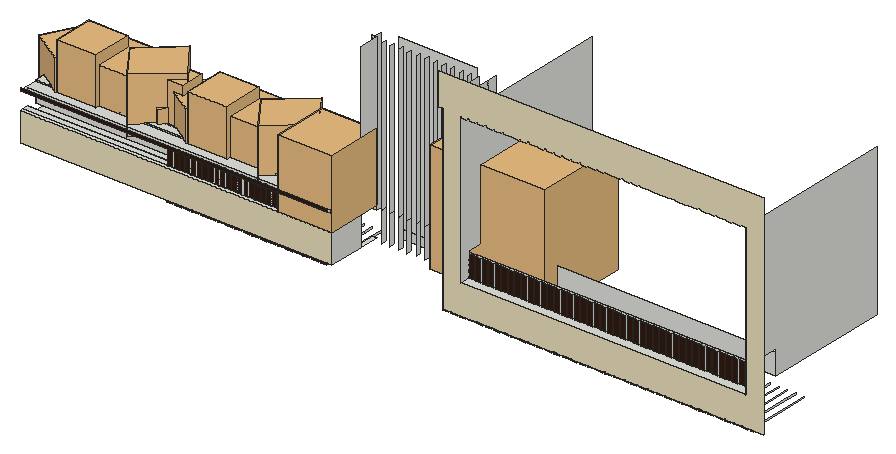
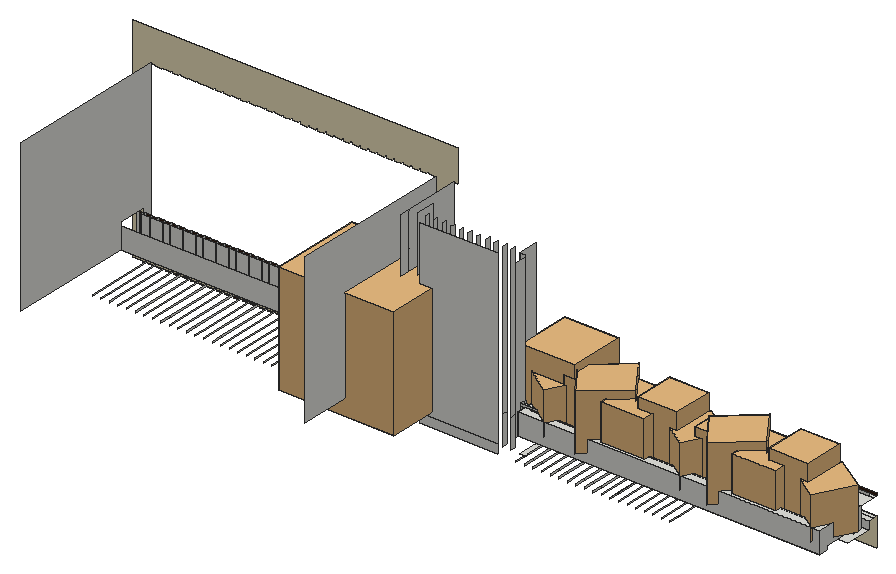
# SketchUp Ruby script. Lengths in inches.
U = 1.inch
M = Sketchup.active_model
def pt(a) = Geom::Point3d.new(a.map { |v| v * U })
def face(e, loops, mat)
  f = e.add_face(loops[0].map { |a| pt(a) })
  loops[1..].each { |l| e.add_face(l.map { |a| pt(a) }).erase! }
  f.material = f.back_material = mat if mat
  f
end
# faces: each face lists its corners as indices into pts; further lists are holes
def faces(e, pts, list, mat = nil) = list.each { |f| face(e, (f[0].is_a?(Array) ? f : [f]).map { |l| l.map { |i| pts[i] } }, mat) }
# xy, xz, yz: faces in a plane at the given z, y or x. An outline is a flat list of corners, or four numbers for a rectangle; further outlines are holes
def ring(l) = l.size == 4 ? [[l[0], l[1]], [l[2], l[1]], [l[2], l[3]], [l[0], l[3]]] : l.each_slice(2).to_a
def flat(e, list, mat, &to3) = list.each { |f| face(e, (f[0].is_a?(Array) ? f : [f]).map { |l| ring(l).map { |u, v| to3.(u, v) } }, mat) }
def xy(e, z, list, mat = nil) = flat(e, list, mat) { |x, y| [x, y, z] }
def xz(e, y, list, mat = nil) = flat(e, list, mat) { |x, z| [x, y, z] }
def yz(e, x, list, mat = nil) = flat(e, list, mat) { |y, z| [x, y, z] }
def lines(e, pts, list) = list.each { |a, b| e.add_line(pt(pts[a]), pt(pts[b])) }
# prism: a flat outline (further loops are holes) pulled along v
def prism(e, loops, v, mat = nil)
  f = face(e, loops, mat); d = Geom::Vector3d.new(v.map { |x| x * U })
  f.pushpull(f.normal.samedirection?(d) ? d.length : -d.length)
end
def box(e, o, s, mat = nil) = prism(e, [[o, [o[0] + s[0], o[1], o[2]], [o[0] + s[0], o[1] + s[1], o[2]], [o[0], o[1] + s[1], o[2]]]], [0, 0, s[2]], mat)
def at(x, y, z, deg = 0) = Geom::Transformation.translation(pt([x, y, z])) * Geom::Transformation.rotation(ORIGIN, Z_AXIS, deg.degrees)
def axes(o, x, y, z) = Geom::Transformation.new([*x, 0, *y, 0, *z, 0, *pt(o).to_a, 1])
def part(name) = M.definitions.add(name)
# library, detail: a bought-in or finely detailed component or shape, given as its bounding box
def library(name, o, s) = part(name).tap { |d| box(d.entities, o, s) }
def detail(e, o, s) = box(e.add_group.entities, o, s)
def put(e, d, t, mat = nil) = e.add_instance(d, t).tap { |i| i.material = mat if mat }
def group(e, t, mat = nil) = e.add_group.tap { |g| g.transformation = t; g.material = mat if mat }.entities
root = M.entities
M.materials.add("Material__1").color = [95, 70, 46]
M.materials.add("[Color D01]").color = [237, 225, 189]
M.materials.add("[Wood Veneer 01]").color = [51, 28, 15]
c1 = library("Areca palm plant",[0,0,0],[49.1,36.6,54.46])
c2 = library("Group\#74",[-84.69,-90.07,-0.36],[176.51,175.13,171.4])
c3 = library("Group20\#1",[-20.81,-17.08,3.79],[39.86,39.43,37.51])
c4 = library("Group\#130",[-7.34,-1.2,0],[38.67,35.81,49.04])
c5 = library("Group38\#2",[14.01,28.44,-23.43],[18.58,18.32,38.89])
c6 = part("Group\#16")
put(c6.entities,c1,axes([-6.2,158.41,6.08],[0.45017,-0.56191,0],[0.66137,0.52986,0],[0,0,0.72]))
put(c6.entities,c1,axes([-6.2,56.6,6.08],[0.45017,-0.56191,0],[0.66137,0.52986,0],[0,0,0.72]))
put(c6.entities,c2,axes([14.93,145.87,6.05],[-0.04961,-0.08593,0],[0.08593,-0.04961,0],[0,0,0.10522]))
put(c6.entities,c3,axes([18.97,79.98,4.77],[0,0.85,0],[-0.85,0,0],[0,0,0.85]))
put(c6.entities,c2,axes([14.93,173.12,6.05],[-0.04961,-0.08593,0],[0.08593,-0.04961,0],[0,0,0.10522]))
put(c6.entities,c2,axes([14.93,193.18,6.05],[-0.04961,-0.08593,0],[0.08593,-0.04961,0],[0,0,0.10522]))
put(c6.entities,c4,axes([24.9375,89.91,8],[0,0.79,0],[-0.79,0,0],[0,0,0.79]))
put(c6.entities,c5,axes([-4.1,-1.15,28.17],[0.8848,0,0],[0,0.94674,0],[0,0,0.85826]))
g1 = group(c6.entities,at(0,0,0))
xy(g1,0,[[0,0,6,234.8],[30,0,36,234.8]])
xy(g1,3,[[6,0,30,234.8]])
xy(g1,7,[[6,5,30,229.8]],"Material__1")
xy(g1,15,[[[0,0,36,234.8],[6,5,30,229.8]]])
xz(g1,0,[[0,0,6,0,6,3,30,3,30,0,36,0,36,15,0,15]])
xz(g1,5,[[6,7,30,15]])
xz(g1,229.8,[[6,7,30,15]])
xz(g1,234.8,[[0,0,0,15,36,15,36,0,30,0,30,3,6,3,6,0]])
yz(g1,0,[[0,0,234.8,15]])
yz(g1,6,[[0,0,234.8,3],[5,7,229.8,15]])
yz(g1,30,[[0,0,234.8,3],[5,7,229.8,15]])
yz(g1,36,[[0,0,234.8,15]])
put(c6.entities,c2,axes([14.93,91.37,6.05],[-0.04961,-0.08593,0],[0.08593,-0.04961,0],[0,0,0.10522]))
put(c6.entities,c2,axes([14.93,44.05,6.05],[-0.04961,-0.08593,0],[0.08593,-0.04961,0],[0,0,0.10522]))
put(c6.entities,c4,axes([24.9375,191.72,8],[0,0.79,0],[-0.79,0,0],[0,0,0.79]))
put(c6.entities,c5,axes([-4.1,100.66,28.17],[0.8848,0,0],[0,0.94674,0],[0,0,0.85826]))
put(c6.entities,c2,axes([17.19,15.79,6.07],[-0.08133,-0.14087,0],[0.14087,-0.08133,0],[0,0,0.1725]))
put(c6.entities,c2,axes([14.93,71.3,6.05],[-0.04961,-0.08593,0],[0.08593,-0.04961,0],[0,0,0.10522]))
put(c6.entities,c2,axes([17.19,121.23,6.07],[-0.08133,-0.14087,0],[0.14087,-0.08133,0],[0,0,0.1725]))
put(c6.entities,c2,axes([17.19,223.04,6.07],[-0.08133,-0.14087,0],[0.14087,-0.08133,0],[0,0,0.1725]))
put(c6.entities,c3,axes([18.97,181.79,4.77],[0,0.85,0],[-0.85,0,0],[0,0,0.85]))
c7 = library("plant (1)",[-35.72,-28.42,0],[66.31,67.39,84.38])
c8 = library("Round Planter with Plant",[-35.48,-39.77,0],[80.62,63.55,77.875])
xy(root,254.6875,[[1782.56,246.64,1785.93,286.21]])
xy(root,269.0625,[[1567.3,253.58,1567.3,271.8,1769.03,271.8,1769.03,290.02,1776.11,290.02,1776.11,253.58]])
xy(root,275.125,[[1567.3,246.64,1785.93,249.27],[1876.45,246.64,2076.2,246.64,2076.2,255.84,1880.14,255.84,1880.14,253.84,1876.45,253.84],[1567.3,249.27,1782.56,253.58],[1782.56,249.27,1785.93,253.58],[1776.11,253.58,1782.56,290.02],
  [1782.56,253.58,1785.93,286.21],[1876.45,253.84,1880.14,255.47]])
xy(root,287.25,[[1567.3,246.64,1782.56,249.27],[1782.56,246.64,1785.1875,249.27],[1567.3,249.27,1567.3,271.8,1769.03,271.8,1769.03,290.02,1782.56,290.02,1782.56,249.27],[1782.56,249.27,1785.1875,286.21]])
xz(root,246.64,[[1711.81,254.625,1716.56,254.6875],[1782.56,287.25,1785.1875,289.1875]])
xz(root,246.64,[[1567.3,254.6875,1785.93,275.125],[[1863.7,254.6875,2089.125,254.6875,2089.125,403.1875,1861.07,403.1875,1861.07,380.6875,1863.7,380.6875],[1876.45,275.125,1876.45,379.5625,1880.86,379.5625,1880.86,380.6875,1882.45,380.6875,1882.45,379.5625,1886.86,379.5625,1886.86,380.6875,1888.45,380.6875,1888.45,379.5625,1892.86,379.5625,1892.86,380.6875,1894.45,380.6875,1894.45,379.5625,1898.86,379.5625,1898.86,380.6875,1900.45,380.6875,1900.45,379.5625,1904.86,379.5625,1904.86,380.6875,1906.45,380.6875,1906.45,379.5625,1910.86,379.5625,1910.86,380.6875,1912.45,380.6875,1912.45,379.5625,1916.86,379.5625,1916.86,380.6875,1918.45,380.6875,1918.45,379.5625,1922.86,379.5625,1922.86,380.6875,1924.45,380.6875,1924.45,379.5625,1928.86,379.5625,1928.86,380.6875,1930.45,380.6875,1930.45,379.5625,1934.86,379.5625,1934.86,380.6875,1936.45,380.6875,1936.45,379.5625,1940.86,379.5625,1940.86,380.6875,1942.45,380.6875,1942.45,379.5625,1946.86,379.5625,1946.86,380.6875,1948.45,380.6875,1948.45,379.5625,1952.86,379.5625,1952.86,380.6875,1954.45,380.6875,1954.45,379.5625,1958.86,379.5625,1958.86,380.6875,1960.45,380.6875,1960.45,379.5625,1964.86,379.5625,1964.86,380.6875,1966.45,380.6875,1966.45,379.5625,1970.86,379.5625,1970.86,380.6875,1972.45,380.6875,1972.45,380.0625,1976.86,380.0625,1976.86,380.6875,1978.45,380.6875,1978.45,380.0625,1982.86,380.0625,1982.86,380.6875,1984.45,380.6875,1984.45,380.0625,1988.86,380.0625,1988.86,380.6875,1990.45,380.6875,1990.45,380.0625,1994.86,380.0625,1994.86,380.6875,1996.45,380.6875,1996.45,380.0625,2000.86,380.0625,2000.86,380.6875,2002.45,380.6875,2002.45,380.0625,2006.86,380.0625,2006.86,380.6875,2008.45,380.6875,2008.45,380.0625,2012.86,380.0625,2012.86,380.6875,2014.45,380.6875,2014.45,380.0625,2018.86,380.0625,2018.86,380.6875,2020.45,380.6875,2020.45,380.0625,2024.86,380.0625,2024.86,380.6875,2026.45,380.6875,2026.45,380.0625,2030.86,380.0625,2030.86,380.6875,2032.45,380.6875,2032.45,380.0625,2036.86,380.0625,2036.86,380.6875,2038.45,380.6875,2038.45,380.1875,2042.86,380.1875,2042.86,380.6875,2044.45,380.6875,2044.45,380.1875,2048.86,380.1875,2048.86,380.6875,2050.45,380.6875,2050.45,380.1875,2054.86,380.1875,2054.86,380.6875,2056.45,380.6875,2056.45,380.1875,2060.86,380.1875,2060.86,380.6875,2062.45,380.6875,2062.45,380.1875,2066.86,380.1875,2066.86,380.6875,2068.45,380.6875,2068.45,380.1875,2072.86,380.1875,2072.86,380.6875,2076.2,380.6875,2076.2,275.125]]],"[Color D01]")
xz(root,246.64,[[1723.81,253.5625,1728.56,254.6875],[1729.81,253.5625,1734.56,254.6875],[1735.81,253.5625,1740.56,254.6875],[1741.81,253.5625,1746.56,254.6875],[1747.81,253.5625,1752.56,254.6875],
  [1753.81,253.5625,1758.56,254.6875],[1759.81,253.5625,1764.56,254.6875],[1765.81,253.5625,1770.56,254.6875],[1771.81,253.5625,1776.56,254.6875],[1777.81,253.5625,1782.56,254.6875],
  [1711.81,253.875,1716.56,254.625],[1717.81,253.875,1722.56,254.6875],[1669.81,253.9375,1674.56,254.6875],[1675.81,253.9375,1680.56,254.6875],[1681.81,253.9375,1686.56,254.6875],
  [1687.81,253.9375,1692.56,254.6875],[1693.81,253.9375,1698.56,254.6875],[1699.81,253.9375,1704.56,254.6875],[1705.81,253.9375,1710.56,254.6875],[1863.7,253.9375,1868.08,254.6875],
  [1869.7,253.9375,1874.08,254.6875],[1875.7,253.9375,1880.08,254.6875],[1881.7,253.9375,1886.08,254.6875],[1887.7,253.9375,1892.08,254.6875],[1893.7,253.9375,1898.08,254.6875],
  [1899.7,253.9375,1904.08,254.6875],[1905.7,253.9375,1910.08,254.6875],[1911.7,253.9375,1916.08,254.6875],[1917.7,253.9375,1922.08,254.6875],[1923.7,253.9375,1928.08,254.6875],
  [1929.7,253.9375,1934.08,254.6875],[1935.7,253.9375,1940.08,254.6875],[1941.7,253.9375,1946.08,254.6875],[1947.7,253.9375,1952.08,254.6875],[1953.7,253.9375,1958.08,254.6875],
  [1959.7,253.9375,1964.08,254.6875],[1965.7,253.9375,1970.08,254.6875],[1971.7,253.9375,1976.08,254.6875],[1977.7,253.9375,1982.08,254.6875],[1983.7,253.9375,1988.08,254.6875],
  [1989.7,253.9375,1994.08,254.6875],[1995.7,253.9375,2000.08,254.6875],[2001.7,253.9375,2006.08,254.6875],[2007.7,253.9375,2012.08,254.6875],[2013.7,253.9375,2018.08,254.6875],
  [2019.7,253.9375,2024.08,254.6875],[2025.7,253.9375,2030.08,254.6875],[2031.7,253.9375,2036.08,254.6875],[2037.7,253.9375,2042.08,254.6875],[2043.7,253.9375,2048.08,254.6875],
  [2049.7,253.9375,2054.08,254.6875],[2055.7,253.9375,2060.08,254.6875],[2061.7,253.9375,2066.08,254.6875],[2067.7,253.9375,2072.08,254.6875],[2073.7,253.9375,2078.08,254.6875],
  [2079.7,253.9375,2081.89,254.6875],[1567.3,287.25,1782.56,289.1875]],"[Wood Veneer 01]")
xz(root,249.27,[[1672.14,275.125,1672.93,287.25],[1676.2,275.125,1676.99,287.25],[1680.27,275.125,1681.05,287.25],[1684.33,275.125,1685.11,287.25],[1688.39,275.125,1689.18,287.25],
  [1692.45,275.125,1693.24,287.25],[1696.52,275.125,1697.3,287.25],[1700.58,275.125,1701.36,287.25],[1704.64,275.125,1705.43,287.25],[1708.7,275.125,1709.49,287.25],
  [1712.77,275.125,1713.55,287.25],[1716.83,275.125,1717.61,287.25],[1720.89,275.125,1721.68,287.25],[1724.95,275.125,1725.74,287.25],[1729.02,275.125,1729.8,287.25],
  [1733.08,275.125,1733.86,287.25],[1737.14,275.125,1737.93,287.25],[1741.2,275.125,1741.99,287.25],[1745.27,275.125,1746.05,287.25],[1749.33,275.125,1750.11,287.25],
  [1753.39,275.125,1754.18,287.25],[1757.45,275.125,1758.24,287.25],[1761.52,275.125,1762.3,287.25],[1765.58,275.125,1766.36,287.25],[1769.64,275.125,1770.43,287.25],
  [1773.7,275.125,1774.49,287.25],[1777.77,275.125,1778.55,287.25],[1781.83,275.125,1782.56,287.25],[1570.58,287.25,1782.56,289.1875],[1782.56,287.25,1785.1875,289.1875]])
xz(root,249.27,[[1668.86,275.125,1672.14,287.25],[1672.93,275.125,1676.2,287.25],[1676.99,275.125,1680.27,287.25],[1681.05,275.125,1684.33,287.25],[1685.11,275.125,1688.39,287.25],
  [1689.18,275.125,1692.45,287.25],[1693.24,275.125,1696.52,287.25],[1697.3,275.125,1700.58,287.25],[1701.36,275.125,1704.64,287.25],[1705.43,275.125,1708.7,287.25],
  [1709.49,275.125,1712.77,287.25],[1713.55,275.125,1716.83,287.25],[1717.61,275.125,1720.89,287.25],[1721.68,275.125,1724.95,287.25],[1725.74,275.125,1729.02,287.25],
  [1729.8,275.125,1733.08,287.25],[1733.86,275.125,1737.14,287.25],[1737.93,275.125,1741.2,287.25],[1741.99,275.125,1745.27,287.25],[1746.05,275.125,1749.33,287.25],
  [1750.11,275.125,1753.39,287.25],[1754.18,275.125,1757.45,287.25],[1758.24,275.125,1761.52,287.25],[1762.3,275.125,1765.58,287.25],[1766.36,275.125,1769.64,287.25],
  [1770.43,275.125,1773.7,287.25],[1774.49,275.125,1777.77,287.25],[1778.55,275.125,1781.83,287.25]],"[Wood Veneer 01]")
xz(root,253.58,[[1567.3,269.0625,1776.11,275.125]])
xz(root,253.84,[[1876.45,275.125,1880.14,290.375],[1881.07,275.125,1884.76,290.375],[1885.7,275.125,1889.39,290.375],[1890.32,275.125,1894.01,290.375],[1894.95,275.125,1898.64,290.375],
  [1899.57,275.125,1903.26,290.375],[1904.2,275.125,1907.89,290.375],[1908.82,275.125,1912.51,290.375],[1913.45,275.125,1917.14,290.375],[1918.07,275.125,1921.76,290.375],
  [1922.7,275.125,1926.39,290.375],[1927.32,275.125,1931.01,290.375],[1931.95,275.125,1935.64,290.375],[1936.57,275.125,1940.26,290.375],[1941.2,275.125,1944.89,290.375],
  [1945.82,275.125,1949.51,290.375],[1950.45,275.125,1954.14,290.375],[1955.07,275.125,1958.76,290.375],[1959.7,275.125,1963.39,290.375],[1964.32,275.125,1968.01,290.375],
  [1968.95,275.125,1972.64,290.375],[1973.57,275.125,1977.26,290.375],[1978.2,275.125,1981.89,290.375],[1982.82,275.125,1986.51,290.375],[1987.45,275.125,1991.14,290.375],
  [1992.07,275.125,1995.76,290.375],[1996.7,275.125,2000.39,290.375],[2001.32,275.125,2005.01,290.375],[2005.95,275.125,2009.64,290.375],[2010.57,275.125,2014.26,290.375],
  [2015.2,275.125,2018.89,290.375],[2019.82,275.125,2023.51,290.375],[2024.45,275.125,2028.14,290.375],[2029.07,275.125,2032.76,290.375],[2033.7,275.125,2037.39,290.375],
  [2038.32,275.125,2042.01,290.375],[2042.95,275.125,2046.64,290.375],[2047.57,275.125,2051.26,290.375],[2052.2,275.125,2055.89,290.375],[2056.82,275.125,2060.51,290.375],
  [2061.45,275.125,2065.14,290.375],[2066.07,275.125,2069.76,290.375],[2070.7,275.125,2074.39,290.375],[2075.32,275.125,2079.01,290.375]],"[Wood Veneer 01]")
xz(root,255.47,[[1876.45,275.125,1880.14,290.375]])
xz(root,255.84,[[1880.14,275.125,2076.2,290.375]])
xz(root,273.33,[[1876.45,275.125,2076.2,290.375]])
xz(root,286.21,[[1782.56,275.125,1785.93,275.125,1785.93,380.6875,1782.56,380.6875,1782.56,289.1875,1785.1875,289.1875,1785.1875,287.25,1782.56,287.25],[1782.56,287.25,1785.1875,289.1875]])
xz(root,290.02,[[1769.03,269.0625,1769.03,287.25,1782.56,287.25,1782.56,275.125,1776.11,275.125,1776.11,269.0625],[1776.11,269.0625,1782.56,275.125],[1769.03,287.25,1782.56,289.1875]])
xz(root,293.45,[[1795.15,254.6875,1849.87,260.6875],[1795.15,260.6875,1849.87,380.6875]])
yz(root,1674.56,[[246.64,253.9375,286.21,254.6875],[286.21,253.9375,293.45,254.6875]])
yz(root,1680.56,[[246.64,253.9375,286.21,254.6875],[286.21,253.9375,293.45,254.6875]])
yz(root,1686.56,[[246.64,253.9375,286.21,254.6875],[286.21,253.9375,293.45,254.6875]])
yz(root,1692.56,[[246.64,253.9375,286.21,254.6875],[286.21,253.9375,293.45,254.6875]])
yz(root,1698.56,[[246.64,253.9375,286.21,254.6875],[286.21,253.9375,293.45,254.6875]])
yz(root,1704.56,[[246.64,253.9375,286.21,254.6875],[286.21,253.9375,293.45,254.6875]])
yz(root,1710.56,[[246.64,253.9375,286.21,254.6875],[286.21,253.9375,293.45,254.6875]])
yz(root,1716.56,[[246.64,253.875,286.21,254.625],[286.21,253.875,293.45,254.625],[246.64,254.625,286.21,254.6875],[286.21,254.625,293.45,254.6875]])
yz(root,1722.56,[[246.64,253.875,286.21,254.6875],[286.21,253.875,293.45,254.6875]])
yz(root,1728.56,[[246.64,253.5625,286.21,254.6875],[286.21,253.5625,293.45,254.6875]])
yz(root,1734.56,[[246.64,253.5625,286.21,254.6875],[286.21,253.5625,293.45,254.6875]])
yz(root,1740.56,[[246.64,253.5625,286.21,254.6875],[286.21,253.5625,293.45,254.6875]])
yz(root,1746.56,[[246.64,253.5625,286.21,254.6875],[286.21,253.5625,293.45,254.6875]])
yz(root,1752.56,[[246.64,253.5625,286.21,254.6875],[286.21,253.5625,293.45,254.6875]])
yz(root,1758.56,[[246.64,253.5625,286.21,254.6875],[286.21,253.5625,293.45,254.6875]])
yz(root,1764.56,[[246.64,253.5625,286.21,254.6875],[286.21,253.5625,293.45,254.6875]])
yz(root,1769.03,[[271.8,269.0625,290.02,287.25],[271.8,287.25,290.02,289.1875]])
yz(root,1770.56,[[246.64,253.5625,286.21,254.6875],[286.21,253.5625,293.45,254.6875]])
yz(root,1776.11,[[253.58,269.0625,290.02,275.125]])
yz(root,1776.56,[[246.64,253.5625,286.21,254.6875],[286.21,253.5625,293.45,254.6875]])
yz(root,1782.56,[[246.64,253.5625,286.21,254.6875],[286.21,253.5625,293.45,254.6875],[290.02,269.0625,290.02,289.1875,286.21,289.1875,286.21,378.875,293.45,378.875,293.45,269.0625],[249.27,275.125,286.21,287.25],[286.21,275.125,290.02,287.25],
  [246.64,287.25,249.27,289.1875],[249.27,287.25,286.21,289.1875],[286.21,287.25,290.02,289.1875]])
yz(root,1785.1875,[[246.64,287.25,249.27,289.1875],[249.27,287.25,286.21,289.1875]])
yz(root,1785.93,[[246.64,254.6875,271.96,275.125],[271.96,275.125,286.21,380.6875]])
yz(root,1791.93,[[282.52,254.6875,286.21,275.125],[282.52,275.125,286.21,380.6875]])
yz(root,1797.93,[[282.52,254.6875,286.21,275.125],[282.52,275.125,286.21,380.6875]])
yz(root,1803.93,[[282.52,254.6875,286.21,275.125],[282.52,275.125,286.21,380.6875]])
yz(root,1809.93,[[282.52,254.6875,286.21,275.125],[282.52,275.125,286.21,380.6875]])
yz(root,1815.93,[[283.46,254.6875,286.21,275.125],[283.46,275.125,286.21,380.6875]])
yz(root,1821.93,[[283.46,254.6875,286.21,275.125],[283.46,275.125,286.21,380.6875]])
yz(root,1827.93,[[283.46,254.6875,286.21,275.125],[283.46,275.125,286.21,380.6875]])
yz(root,1833.93,[[283.46,254.6875,286.21,275.125],[283.46,275.125,286.21,380.6875]])
yz(root,1839.93,[[283.46,254.6875,286.21,275.125],[283.46,275.125,286.21,380.6875]])
yz(root,1845.93,[[283.46,254.6875,286.21,275.125],[283.46,275.125,286.21,380.6875]])
yz(root,1851.93,[[283.46,254.6875,286.21,275.125],[283.46,275.125,286.21,380.6875]])
yz(root,1857.25,[[272.89,254.6875,286.21,275.125],[272.89,275.125,286.21,380.6875]])
yz(root,1863.7,[[246.64,253.9375,286.21,254.6875],[286.21,253.9375,293.45,254.6875],[246.64,254.6875,286.21,260.6875],[286.21,254.6875,293.45,260.6875],[246.64,260.6875,286.21,380.6875],
  [286.21,260.6875,293.45,380.6875]])
yz(root,1869.7,[[246.64,253.9375,286.21,254.6875],[286.21,253.9375,293.45,254.6875]])
yz(root,1875.7,[[246.64,253.9375,286.21,254.6875],[286.21,253.9375,293.45,254.6875]])
yz(root,1876.45,[[246.64,275.125,253.84,275.125,253.84,290.375,253.22,290.375,253.22,292.5625,273.33,292.5625,273.33,275.125,361.27,275.125,361.27,379.5625,246.64,379.5625],[253.84,275.125,255.47,290.375]])
yz(root,1880.14,[[253.84,275.125,255.47,290.375],[255.47,275.125,255.84,290.375]])
yz(root,1881.7,[[246.64,253.9375,286.21,254.6875],[286.21,253.9375,293.45,254.6875]])
yz(root,1884.76,[[253.84,275.125,255.47,290.375]])
yz(root,1887.7,[[246.64,253.9375,286.21,254.6875],[286.21,253.9375,293.45,254.6875]])
yz(root,1889.39,[[253.84,275.125,255.47,290.375]])
yz(root,1893.7,[[246.64,253.9375,286.21,254.6875],[286.21,253.9375,293.45,254.6875]])
yz(root,1894.01,[[253.84,275.125,255.47,290.375]])
yz(root,1898.64,[[253.84,275.125,255.47,290.375]])
yz(root,1899.7,[[246.64,253.9375,286.21,254.6875],[286.21,253.9375,293.45,254.6875]])
yz(root,1903.26,[[253.84,275.125,255.47,290.375]])
yz(root,1905.7,[[246.64,253.9375,286.21,254.6875],[286.21,253.9375,293.45,254.6875]])
yz(root,1907.89,[[253.84,275.125,255.47,290.375]])
yz(root,1911.7,[[246.64,253.9375,286.21,254.6875],[286.21,253.9375,293.45,254.6875]])
yz(root,1912.51,[[253.84,275.125,255.47,290.375]])
yz(root,1917.14,[[253.84,275.125,255.47,290.375]])
yz(root,1917.7,[[246.64,253.9375,286.21,254.6875],[286.21,253.9375,293.45,254.6875]])
yz(root,1921.76,[[253.84,275.125,255.47,290.375]])
yz(root,1923.7,[[246.64,253.9375,286.21,254.6875],[286.21,253.9375,293.45,254.6875]])
yz(root,1926.39,[[253.84,275.125,255.47,290.375]])
yz(root,1929.7,[[246.64,253.9375,286.21,254.6875],[286.21,253.9375,293.45,254.6875]])
yz(root,1931.01,[[253.84,275.125,255.47,290.375]])
yz(root,1935.64,[[253.84,275.125,255.47,290.375]])
yz(root,1935.7,[[246.64,253.9375,286.21,254.6875],[286.21,253.9375,293.45,254.6875]])
yz(root,1940.26,[[253.84,275.125,255.47,290.375]])
yz(root,1941.7,[[246.64,253.9375,286.21,254.6875],[286.21,253.9375,293.45,254.6875]])
yz(root,1944.89,[[253.84,275.125,255.47,290.375]])
yz(root,1947.7,[[246.64,253.9375,286.21,254.6875],[286.21,253.9375,293.45,254.6875]])
yz(root,1949.51,[[253.84,275.125,255.47,290.375]])
yz(root,1953.7,[[246.64,253.9375,286.21,254.6875],[286.21,253.9375,293.45,254.6875]])
yz(root,1954.14,[[253.84,275.125,255.47,290.375]])
yz(root,1958.76,[[253.84,275.125,255.47,290.375]])
yz(root,1959.7,[[246.64,253.9375,286.21,254.6875],[286.21,253.9375,293.45,254.6875]])
yz(root,1963.39,[[253.84,275.125,255.47,290.375]])
yz(root,1965.7,[[246.64,253.9375,286.21,254.6875],[286.21,253.9375,293.45,254.6875]])
yz(root,1968.01,[[253.84,275.125,255.47,290.375]])
yz(root,1971.7,[[246.64,253.9375,286.21,254.6875],[286.21,253.9375,293.45,254.6875]])
yz(root,1972.64,[[253.84,275.125,255.47,290.375]])
yz(root,1977.26,[[253.84,275.125,255.47,290.375]])
yz(root,1977.7,[[246.64,253.9375,286.21,254.6875],[286.21,253.9375,293.45,254.6875]])
yz(root,1981.89,[[253.84,275.125,255.47,290.375]])
yz(root,1983.7,[[246.64,253.9375,286.21,254.6875],[286.21,253.9375,293.45,254.6875]])
yz(root,1986.51,[[253.84,275.125,255.47,290.375]])
yz(root,1989.7,[[246.64,253.9375,286.21,254.6875],[286.21,253.9375,293.45,254.6875]])
yz(root,1991.14,[[253.84,275.125,255.47,290.375]])
yz(root,1995.7,[[246.64,253.9375,286.21,254.6875],[286.21,253.9375,293.45,254.6875]])
yz(root,1995.76,[[253.84,275.125,255.47,290.375]])
yz(root,2000.39,[[253.84,275.125,255.47,290.375]])
yz(root,2001.7,[[246.64,253.9375,286.21,254.6875],[286.21,253.9375,293.45,254.6875]])
yz(root,2005.01,[[253.84,275.125,255.47,290.375]])
yz(root,2007.7,[[246.64,253.9375,286.21,254.6875],[286.21,253.9375,293.45,254.6875]])
yz(root,2009.64,[[253.84,275.125,255.47,290.375]])
yz(root,2013.7,[[246.64,253.9375,286.21,254.6875],[286.21,253.9375,293.45,254.6875]])
yz(root,2014.26,[[253.84,275.125,255.47,290.375]])
yz(root,2018.89,[[253.84,275.125,255.47,290.375]])
yz(root,2019.7,[[246.64,253.9375,286.21,254.6875],[286.21,253.9375,293.45,254.6875]])
yz(root,2023.51,[[253.84,275.125,255.47,290.375]])
yz(root,2025.7,[[246.64,253.9375,286.21,254.6875],[286.21,253.9375,293.45,254.6875]])
yz(root,2028.14,[[253.84,275.125,255.47,290.375]])
yz(root,2031.7,[[246.64,253.9375,286.21,254.6875],[286.21,253.9375,293.45,254.6875]])
yz(root,2032.76,[[253.84,275.125,255.47,290.375]])
yz(root,2037.39,[[253.84,275.125,255.47,290.375]])
yz(root,2037.7,[[246.64,253.9375,286.21,254.6875],[286.21,253.9375,293.45,254.6875]])
yz(root,2042.01,[[253.84,275.125,255.47,290.375]])
yz(root,2043.7,[[246.64,253.9375,286.21,254.6875],[286.21,253.9375,293.45,254.6875]])
yz(root,2046.64,[[253.84,275.125,255.47,290.375]])
yz(root,2049.7,[[246.64,253.9375,286.21,254.6875],[286.21,253.9375,293.45,254.6875]])
yz(root,2051.26,[[253.84,275.125,255.47,290.375]])
yz(root,2055.7,[[246.64,253.9375,286.21,254.6875],[286.21,253.9375,293.45,254.6875]])
yz(root,2055.89,[[253.84,275.125,255.47,290.375]])
yz(root,2060.51,[[253.84,275.125,255.47,290.375]])
yz(root,2061.7,[[246.64,253.9375,286.21,254.6875],[286.21,253.9375,293.45,254.6875]])
yz(root,2065.14,[[253.84,275.125,255.47,290.375]])
yz(root,2067.7,[[246.64,253.9375,286.21,254.6875],[286.21,253.9375,293.45,254.6875]])
yz(root,2069.76,[[253.84,275.125,255.47,290.375]])
yz(root,2073.7,[[246.64,253.9375,286.21,254.6875],[286.21,253.9375,293.45,254.6875]])
yz(root,2074.39,[[253.84,275.125,255.47,290.375]])
yz(root,2076.2,[[246.64,275.125,246.64,380.6875,361.27,380.6875,361.27,275.125,273.33,275.125,273.33,292.5625,253.22,292.5625,253.22,290.375,255.84,290.375,255.84,275.125]])
yz(root,2079.01,[[253.84,275.125,255.47,290.375]])
yz(root,2079.7,[[246.64,253.9375,286.21,254.6875],[286.21,253.9375,293.45,254.6875]])
put(root,c6,axes([1778.89,260.97,273.05],[0,1,0],[-0.9045,0,0],[0,0,1]))
put(root,c7,axes([1768.5,262.85,275.125],[0.57,0,0],[0,0.57,0],[0,0,0.57]))
put(root,c8,at(1876.93,303,264.4375))
